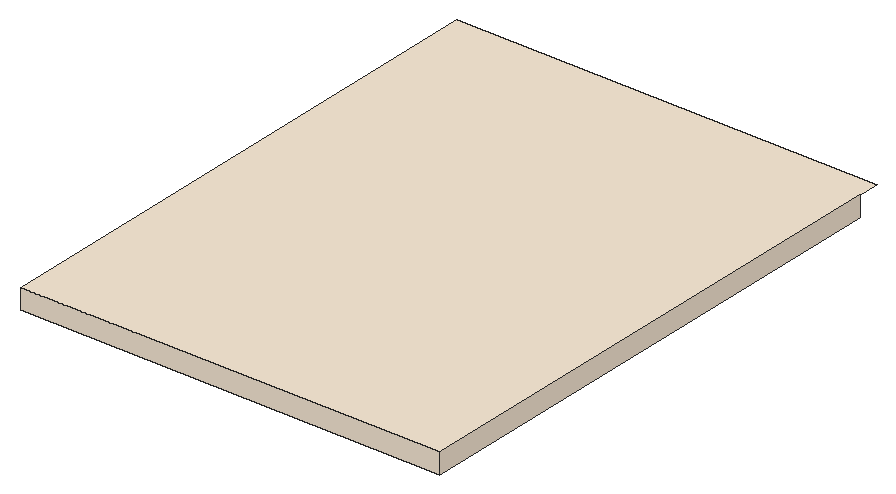
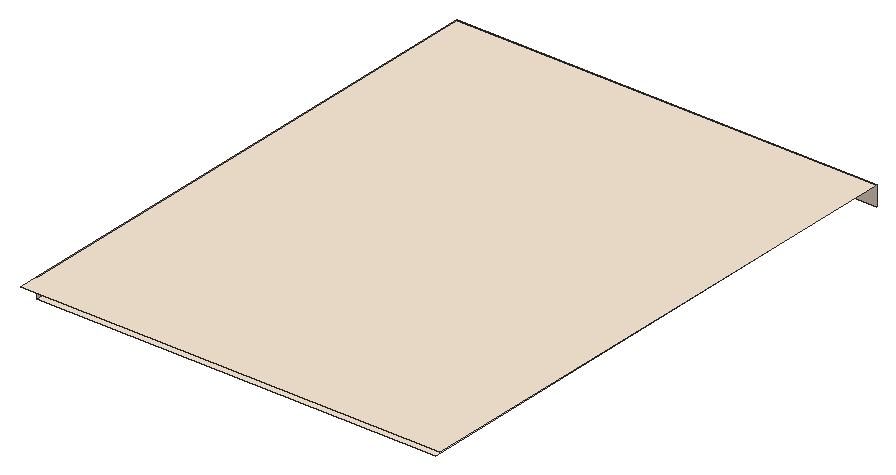
# SketchUp Ruby script. Lengths in inches.
U = 1.inch
M = Sketchup.active_model
def pt(a) = Geom::Point3d.new(a.map { |v| v * U })
def face(e, loops, mat)
  f = e.add_face(loops[0].map { |a| pt(a) })
  loops[1..].each { |l| e.add_face(l.map { |a| pt(a) }).erase! }
  f.material = f.back_material = mat if mat
  f
end
# faces: each face lists its corners as indices into pts; further lists are holes
def faces(e, pts, list, mat = nil) = list.each { |f| face(e, (f[0].is_a?(Array) ? f : [f]).map { |l| l.map { |i| pts[i] } }, mat) }
# xy, xz, yz: faces in a plane at the given z, y or x. An outline is a flat list of corners, or four numbers for a rectangle; further outlines are holes
def ring(l) = l.size == 4 ? [[l[0], l[1]], [l[2], l[1]], [l[2], l[3]], [l[0], l[3]]] : l.each_slice(2).to_a
def flat(e, list, mat, &to3) = list.each { |f| face(e, (f[0].is_a?(Array) ? f : [f]).map { |l| ring(l).map { |u, v| to3.(u, v) } }, mat) }
def xy(e, z, list, mat = nil) = flat(e, list, mat) { |x, y| [x, y, z] }
def xz(e, y, list, mat = nil) = flat(e, list, mat) { |x, z| [x, y, z] }
def yz(e, x, list, mat = nil) = flat(e, list, mat) { |y, z| [x, y, z] }
def lines(e, pts, list) = list.each { |a, b| e.add_line(pt(pts[a]), pt(pts[b])) }
# prism: a flat outline (further loops are holes) pulled along v
def prism(e, loops, v, mat = nil)
  f = face(e, loops, mat); d = Geom::Vector3d.new(v.map { |x| x * U })
  f.pushpull(f.normal.samedirection?(d) ? d.length : -d.length)
end
def box(e, o, s, mat = nil) = prism(e, [[o, [o[0] + s[0], o[1], o[2]], [o[0] + s[0], o[1] + s[1], o[2]], [o[0], o[1] + s[1], o[2]]]], [0, 0, s[2]], mat)
def at(x, y, z, deg = 0) = Geom::Transformation.translation(pt([x, y, z])) * Geom::Transformation.rotation(ORIGIN, Z_AXIS, deg.degrees)
def axes(o, x, y, z) = Geom::Transformation.new([*x, 0, *y, 0, *z, 0, *pt(o).to_a, 1])
def part(name) = M.definitions.add(name)
# library, detail: a bought-in or finely detailed component or shape, given as its bounding box
def library(name, o, s) = part(name).tap { |d| box(d.entities, o, s) }
def detail(e, o, s) = box(e.add_group.entities, o, s)
def put(e, d, t, mat = nil) = e.add_instance(d, t).tap { |i| i.material = mat if mat }
def group(e, t, mat = nil) = e.add_group.tap { |g| g.transformation = t; g.material = mat if mat }.entities
root = M.entities
M.materials.add("[0028_AntiqueWhite]").color = [250, 235, 215]
M.materials.add("[Granite Light Gray]").color = [149, 148, 144]
xy(root,231.4,[[[30.25,60.67,29.63,60.78,29.02,60.95,28.43,61.19,27.87,61.49,27.35,61.84,26.86,62.24,26.41,62.6875,26.01,63.18,25.67,63.71,25.38,64.27,25.15,64.86,24.98,65.47,24.98,232.53,25.03,233.34,25.1875,234.13,25.45,234.9,25.81,235.62,26.25,236.29,26.79,236.9,27.39,237.43,28.07,237.88,28.79,238.24,29.55,238.5,30.35,238.66,31.15,238.71,182.85,238.71,183.6,238.55,184.33,238.3,185.02,237.96,185.67,237.55,186.27,237.0625,186.81,236.51,187.27,235.9,187.66,235.23,187.97,234.53,188.2,233.79,188.33,233.03,188.38,232.26,188.38,66.48,188.2,65.68,187.93,64.92,187.57,64.1875,187.13,63.5,186.61,62.875,186.02,62.31,185.37,61.83,184.67,61.42,183.92,61.09,183.14,60.86,182.34,60.71,181.53,60.67],[30.47,63.11,181.46,63.11,182.06,63.14,182.58,63.24,183.08,63.39,183.5625,63.6,184.02,63.86,184.4375,64.18,184.82,64.54,185.15,64.95,185.44,65.39,185.67,65.86,185.85,66.36,185.93,66.75,185.93,232.19,185.9,232.74,185.82,233.22,185.68,233.68,185.48,234.12,185.24,234.53,184.95,234.92,184.61,235.26,184.24,235.57,183.83,235.82,183.4,236.03,182.95,236.1875,182.59,236.27,31.15,236.27,30.67,236.23,30.1875,236.14,29.72,235.98,29.29,235.77,28.88,235.49,28.51,235.17,28.19,234.81,27.92,234.4,27.71,233.96,27.55,233.5,27.45,233.02,27.42,232.53,27.42,65.81,27.47,65.64,27.61,65.28,27.78,64.9375,27.99,64.62,28.23,64.32,28.5,64.05,28.8,63.8,29.12,63.59,29.46,63.41,29.82,63.27,30.1875,63.16]]],"[Granite Light Gray]")
xy(root,232.34,[[[37.8125,67.21,37.07,67.33,36.34,67.53,35.63,67.81,34.96,68.15,34.33,68.57,33.74,69.04,33.21,69.58,32.74,70.17,32.33,70.8,31.99,71.48,31.72,72.18,31.52,72.91,31.52,227.33,31.66,227.92,31.86,228.49,32.12,229.04,32.42,229.5625,32.78,230.05,33.19,230.5,33.64,230.9,34.125,231.26,34.65,231.57,35.2,231.83,35.77,232.02,36.36,232.16,177.3125,232.16,177.86,232.03,178.4,231.85,178.91,231.61,179.4,231.33,179.86,230.99,180.28,230.61,180.66,230.19,181,229.73,181.28,229.25,181.52,228.73,181.7,228.19,181.83,227.64,181.83,71.75,181.71,71.13,181.51,70.53,181.24,69.97,180.91,69.43,180.52,68.94,180.07,68.5,179.57,68.12,179.03,67.8,178.46,67.54,177.86,67.36,177.24,67.25,176.61,67.21],[37.91,68.4,176.58,68.4,177.1,68.43,177.58,68.52,178.04,68.66,178.49,68.86,178.9,69.11,179.29,69.4,179.64,69.74,179.94,70.12,180.2,70.53,180.4,70.97,180.56,71.4375,180.64,71.87,180.64,227.51,180.56,227.87,180.41,228.29,180.23,228.69,180,229.08,179.74,229.4375,179.4375,229.77,179.11,230.07,178.75,230.33,178.36,230.56,177.96,230.75,177.53,230.89,177.18,230.97,36.5,230.97,36.1,230.88,35.64,230.72,35.2,230.52,34.78,230.27,34.39,229.98,34.03,229.66,33.71,229.3,33.42,228.9,33.17,228.49,32.97,228.04,32.81,227.59,32.71,227.19,32.71,73.07,32.85,72.55,33.08,71.96,33.36,71.4,33.7,70.87,34.1,70.375,34.54,69.93,35.03,69.53,35.5625,69.18,36.12,68.89,36.71,68.66,37.32,68.5]]],"[Granite Light Gray]")
xy(root,233.77,[[24.97,7.66,24.05,7.72,23.14,7.9,22.26,8.2,21.43,8.61,20.66,9.12,19.96,9.73,19.35,10.43,18.84,11.2,18.43,12.03,18.13,12.91,17.95,13.82,17.89,14.74,17.89,31.67,17.94,32.53,18.11,33.38,18.39,34.2,18.77,34.97,19.25,35.69,19.82,36.33,20.47,36.9,21.18,37.38,21.95,37.76,22.77,38.04,23.62,38.21,24.48,38.26,190.49,38.26,191.11,38.14,191.71,37.96,192.29,37.71,192.84,37.4,193.35,37.03,193.82,36.61,194.24,36.14,194.61,35.63,194.92,35.08,195.16,34.5,195.35,33.9,195.47,33.28,195.47,12.37,195.34,11.73,195.14,11.11,194.86,10.52,194.52,9.97,194.11,9.46,193.64,9,193.125,8.6,192.5625,8.27,191.97,8,191.34,7.8125,190.7,7.7,190.05,7.66]],"[Granite Light Gray]")
xy(root,234.21,[[[10.23,45.92,203.125,253.46],[30.25,60.67,181.53,60.67,182.34,60.71,183.14,60.86,183.92,61.09,184.67,61.42,185.37,61.83,186.02,62.31,186.61,62.875,187.13,63.5,187.57,64.1875,187.93,64.92,188.2,65.68,188.38,66.48,188.38,232.26,188.33,233.03,188.2,233.79,187.97,234.53,187.66,235.23,187.27,235.9,186.81,236.51,186.27,237.0625,185.67,237.55,185.02,237.96,184.33,238.3,183.6,238.55,182.85,238.71,31.15,238.71,30.35,238.66,29.55,238.5,28.79,238.24,28.07,237.88,27.39,237.43,26.79,236.9,26.25,236.29,25.81,235.62,25.45,234.9,25.1875,234.13,25.03,233.34,24.98,232.53,24.98,65.47,25.15,64.86,25.38,64.27,25.67,63.71,26.01,63.18,26.41,62.6875,26.86,62.24,27.35,61.84,27.87,61.49,28.43,61.19,29.02,60.95,29.63,60.78]],[37.91,68.4,37.32,68.5,36.71,68.66,36.12,68.89,35.5625,69.18,35.03,69.53,34.54,69.93,34.1,70.375,33.7,70.87,33.36,71.4,33.08,71.96,32.85,72.55,32.71,73.07,32.71,227.19,32.81,227.59,32.97,228.04,33.17,228.49,33.42,228.9,33.71,229.3,34.03,229.66,34.39,229.98,34.78,230.27,35.2,230.52,35.64,230.72,36.1,230.88,36.5,230.97,177.18,230.97,177.53,230.89,177.96,230.75,178.36,230.56,178.75,230.33,179.11,230.07,179.4375,229.77,179.74,229.4375,180,229.08,180.23,228.69,180.41,228.29,180.56,227.87,180.64,227.51,180.64,71.87,180.56,71.4375,180.4,70.97,180.2,70.53,179.94,70.12,179.64,69.74,179.29,69.4,178.9,69.11,178.49,68.86,178.04,68.66,177.58,68.52,177.1,68.43,176.58,68.4]],"[0028_AntiqueWhite]")
xy(root,234.21,[[[30.47,63.11,30.1875,63.16,29.82,63.27,29.46,63.41,29.12,63.59,28.8,63.8,28.5,64.05,28.23,64.32,27.99,64.62,27.78,64.9375,27.61,65.28,27.47,65.64,27.42,65.81,27.42,232.53,27.45,233.02,27.55,233.5,27.71,233.96,27.92,234.4,28.19,234.81,28.51,235.17,28.88,235.49,29.29,235.77,29.72,235.98,30.1875,236.14,30.67,236.23,31.15,236.27,182.59,236.27,182.95,236.1875,183.4,236.03,183.83,235.82,184.24,235.57,184.61,235.26,184.95,234.92,185.24,234.53,185.48,234.12,185.68,233.68,185.82,233.22,185.9,232.74,185.93,232.19,185.93,66.75,185.85,66.36,185.67,65.86,185.44,65.39,185.15,64.95,184.82,64.54,184.4375,64.18,184.02,63.86,183.5625,63.6,183.08,63.39,182.58,63.24,182.06,63.14,181.46,63.11],[37.8125,67.21,176.61,67.21,177.24,67.25,177.86,67.36,178.46,67.54,179.03,67.8,179.57,68.12,180.07,68.5,180.52,68.94,180.91,69.43,181.24,69.97,181.51,70.53,181.71,71.13,181.83,71.75,181.83,227.64,181.7,228.19,181.52,228.73,181.28,229.25,181,229.73,180.66,230.19,180.28,230.61,179.86,230.99,179.4,231.33,178.91,231.61,178.4,231.85,177.86,232.03,177.3125,232.16,36.36,232.16,35.77,232.02,35.2,231.83,34.65,231.57,34.125,231.26,33.64,230.9,33.19,230.5,32.78,230.05,32.42,229.5625,32.12,229.04,31.86,228.49,31.66,227.92,31.52,227.33,31.52,72.91,31.72,72.18,31.99,71.48,32.33,70.8,32.74,70.17,33.21,69.58,33.74,69.04,34.33,68.57,34.96,68.15,35.63,67.81,36.34,67.53,37.07,67.33]]],"[Granite Light Gray]")
xy(root,243.9,[[0,0,203.125,263.6875]],"[0028_AntiqueWhite]")
xz(root,0,[[0,234.21,203.125,243.9]],"[0028_AntiqueWhite]")
xz(root,60.67,[[30.25,231.4,181.53,234.21]],"[Granite Light Gray]")
xz(root,63.11,[[30.47,231.4,181.46,234.21]],"[Granite Light Gray]")
xz(root,67.21,[[37.8125,232.34,176.61,234.21]],"[0028_AntiqueWhite]")
xz(root,68.4,[[37.91,232.34,176.58,234.21]],"[Granite Light Gray]")
xz(root,230.97,[[36.5,232.34,177.18,234.21]],"[Granite Light Gray]")
xz(root,232.16,[[36.36,232.34,177.3125,234.21]],"[Granite Light Gray]")
xz(root,236.27,[[31.15,231.4,182.59,234.21]],"[Granite Light Gray]")
xz(root,238.71,[[31.15,231.4,182.85,234.21]],"[Granite Light Gray]")
yz(root,24.98,[[65.47,231.4,232.53,234.21]],"[0028_AntiqueWhite]")
yz(root,27.42,[[65.81,231.4,232.53,234.21]],"[Granite Light Gray]")
yz(root,31.52,[[72.91,232.34,227.33,234.21]],"[0028_AntiqueWhite]")
yz(root,32.71,[[73.07,232.34,227.19,234.21]],"[Granite Light Gray]")
yz(root,180.64,[[71.87,232.34,227.51,234.21]],"[0028_AntiqueWhite]")
yz(root,181.83,[[71.75,232.34,227.64,234.21]],"[Granite Light Gray]")
yz(root,185.93,[[66.75,231.4,232.19,234.21]],"[0028_AntiqueWhite]")
yz(root,188.38,[[66.48,231.4,232.26,234.21]],"[Granite Light Gray]")
yz(root,203.125,[[0,234.21,253.46,243.9]],"[0028_AntiqueWhite]")
p = [[30.25,60.67,234.21],[29.63,60.78,234.21],[29.63,60.78,231.4],[30.25,60.67,231.4],[182.34,60.71,234.21],[181.53,60.67,234.21],
  [181.53,60.67,231.4],[182.34,60.71,231.4],[183.14,60.86,234.21],[183.14,60.86,231.4],[29.02,60.95,234.21],[29.02,60.95,231.4],
  [183.92,61.09,234.21],[183.92,61.09,231.4],[28.43,61.19,234.21],[28.43,61.19,231.4],[184.67,61.42,234.21],[184.67,61.42,231.4],
  [27.87,61.49,234.21],[27.87,61.49,231.4],[185.37,61.83,234.21],[185.37,61.83,231.4],[27.35,61.84,234.21],[27.35,61.84,231.4],
  [26.86,62.24,234.21],[26.86,62.24,231.4],[186.02,62.31,234.21],[186.02,62.31,231.4],[26.41,62.6875,234.21],[26.41,62.6875,231.4],
  [186.61,62.875,234.21],[186.61,62.875,231.4],[26.01,63.18,234.21],[26.01,63.18,231.4],[187.13,63.5,234.21],[187.13,63.5,231.4],
  [30.1875,63.16,234.21],[30.47,63.11,234.21],[30.47,63.11,231.4],[30.1875,63.16,231.4],[181.46,63.11,234.21],[182.06,63.14,234.21],
  [182.06,63.14,231.4],[181.46,63.11,231.4],[182.58,63.24,234.21],[182.58,63.24,231.4],[25.67,63.71,234.21],[25.67,63.71,231.4],
  [29.82,63.27,234.21],[29.82,63.27,231.4],[183.08,63.39,234.21],[183.08,63.39,231.4],[29.46,63.41,234.21],[29.46,63.41,231.4],
  [29.12,63.59,234.21],[29.12,63.59,231.4],[183.5625,63.6,234.21],[183.5625,63.6,231.4],[187.57,64.1875,234.21],[187.57,64.1875,231.4],
  [28.8,63.8,234.21],[28.8,63.8,231.4],[184.02,63.86,234.21],[184.02,63.86,231.4],[25.38,64.27,234.21],[25.38,64.27,231.4],
  [28.5,64.05,234.21],[28.5,64.05,231.4],[184.4375,64.18,234.21],[184.4375,64.18,231.4],[28.23,64.32,234.21],[28.23,64.32,231.4],
  [184.82,64.54,234.21],[184.82,64.54,231.4],[187.93,64.92,234.21],[187.93,64.92,231.4],[25.15,64.86,234.21],[25.15,64.86,231.4],
  [27.99,64.62,234.21],[27.99,64.62,231.4],[185.15,64.95,234.21],[185.15,64.95,231.4],[27.78,64.9375,234.21],[27.78,64.9375,231.4],
  [24.98,65.47,234.21],[24.98,65.47,231.4],[27.61,65.28,234.21],[27.61,65.28,231.4],[185.44,65.39,234.21],[185.44,65.39,231.4],
  [188.2,65.68,234.21],[188.2,65.68,231.4],[27.47,65.64,234.21],[27.47,65.64,231.4],[185.67,65.86,234.21],[185.67,65.86,231.4],
  [27.42,65.81,234.21],[27.42,65.81,231.4],[188.38,66.48,234.21],[188.38,66.48,231.4],[185.85,66.36,234.21],[185.85,66.36,231.4],
  [185.93,66.75,234.21],[185.93,66.75,231.4],[185.93,232.19,234.21],[185.9,232.74,234.21],[185.9,232.74,231.4],[185.93,232.19,231.4],
  [188.33,233.03,234.21],[188.38,232.26,234.21],[188.38,232.26,231.4],[188.33,233.03,231.4],[24.98,232.53,234.21],[25.03,233.34,234.21],
  [25.03,233.34,231.4],[24.98,232.53,231.4],[27.45,233.02,234.21],[27.42,232.53,234.21],[27.42,232.53,231.4],[27.45,233.02,231.4],
  [185.82,233.22,234.21],[185.82,233.22,231.4],[27.55,233.5,234.21],[27.55,233.5,231.4],[188.2,233.79,234.21],[188.2,233.79,231.4],
  [185.68,233.68,234.21],[185.68,233.68,231.4],[25.1875,234.13,234.21],[25.1875,234.13,231.4],[27.71,233.96,234.21],[27.71,233.96,231.4],
  [185.48,234.12,234.21],[185.48,234.12,231.4],[187.97,234.53,234.21],[187.97,234.53,231.4],[27.92,234.4,234.21],[27.92,234.4,231.4],
  [25.45,234.9,234.21],[25.45,234.9,231.4],[185.24,234.53,234.21],[185.24,234.53,231.4],[28.19,234.81,234.21],[28.19,234.81,231.4],
  [184.95,234.92,234.21],[184.95,234.92,231.4],[187.66,235.23,234.21],[187.66,235.23,231.4],[28.51,235.17,234.21],[28.51,235.17,231.4],
  [25.81,235.62,234.21],[25.81,235.62,231.4],[184.61,235.26,234.21],[184.61,235.26,231.4],[28.88,235.49,234.21],[28.88,235.49,231.4],
  [187.27,235.9,234.21],[187.27,235.9,231.4],[184.24,235.57,234.21],[184.24,235.57,231.4],[29.29,235.77,234.21],[29.29,235.77,231.4],
  [26.25,236.29,234.21],[26.25,236.29,231.4],[183.83,235.82,234.21],[183.83,235.82,231.4],[29.72,235.98,234.21],[29.72,235.98,231.4],
  [183.4,236.03,234.21],[183.4,236.03,231.4],[186.81,236.51,234.21],[186.81,236.51,231.4],[30.1875,236.14,234.21],[30.1875,236.14,231.4],
  [182.95,236.1875,234.21],[182.95,236.1875,231.4],[30.67,236.23,234.21],[30.67,236.23,231.4],[31.15,236.27,234.21],[31.15,236.27,231.4],
  [182.59,236.27,234.21],[182.59,236.27,231.4],[26.79,236.9,234.21],[26.79,236.9,231.4],[186.27,237.0625,234.21],[186.27,237.0625,231.4],
  [27.39,237.43,234.21],[27.39,237.43,231.4],[185.67,237.55,234.21],[185.67,237.55,231.4],[28.07,237.88,234.21],[28.07,237.88,231.4],
  [185.02,237.96,234.21],[185.02,237.96,231.4],[28.79,238.24,234.21],[28.79,238.24,231.4],[184.33,238.3,234.21],[184.33,238.3,231.4],
  [29.55,238.5,234.21],[29.55,238.5,231.4],[183.6,238.55,234.21],[183.6,238.55,231.4],[30.35,238.66,234.21],[30.35,238.66,231.4],
  [182.85,238.71,234.21],[182.85,238.71,231.4],[31.15,238.71,234.21],[31.15,238.71,231.4],[37.8125,67.21,234.21],[37.07,67.33,234.21],
  [37.07,67.33,232.34],[37.8125,67.21,232.34],[177.24,67.25,234.21],[176.61,67.21,234.21],[176.61,67.21,232.34],[177.24,67.25,232.34],
  [177.86,67.36,234.21],[177.86,67.36,232.34],[36.34,67.53,234.21],[36.34,67.53,232.34],[178.46,67.54,234.21],[178.46,67.54,232.34],
  [35.63,67.81,234.21],[35.63,67.81,232.34],[179.03,67.8,234.21],[179.03,67.8,232.34],[34.96,68.15,234.21],[34.96,68.15,232.34],
  [179.57,68.12,234.21],[179.57,68.12,232.34],[180.07,68.5,234.21],[180.07,68.5,232.34],[34.33,68.57,234.21],[34.33,68.57,232.34],
  [37.32,68.5,234.21],[37.91,68.4,234.21],[37.91,68.4,232.34],[37.32,68.5,232.34],[176.58,68.4,234.21],[177.1,68.43,234.21],
  [177.1,68.43,232.34],[176.58,68.4,232.34],[177.58,68.52,234.21],[177.58,68.52,232.34],[36.71,68.66,234.21],[36.71,68.66,232.34],
  [178.04,68.66,234.21],[178.04,68.66,232.34],[180.52,68.94,234.21],[180.52,68.94,232.34],[33.74,69.04,234.21],[33.74,69.04,232.34],
  [36.12,68.89,234.21],[36.12,68.89,232.34],[178.49,68.86,234.21],[178.49,68.86,232.34],[35.5625,69.18,234.21],[35.5625,69.18,232.34],
  [178.9,69.11,234.21],[178.9,69.11,232.34],[180.91,69.43,234.21],[180.91,69.43,232.34],[33.21,69.58,234.21],[33.21,69.58,232.34],
  [179.29,69.4,234.21],[179.29,69.4,232.34],[35.03,69.53,234.21],[35.03,69.53,232.34],[179.64,69.74,234.21],[179.64,69.74,232.34],
  [181.24,69.97,234.21],[181.24,69.97,232.34],[34.54,69.93,234.21],[34.54,69.93,232.34],[32.74,70.17,234.21],[32.74,70.17,232.34],
  [179.94,70.12,234.21],[179.94,70.12,232.34],[34.1,70.375,234.21],[34.1,70.375,232.34],[181.51,70.53,234.21],[181.51,70.53,232.34],
  [180.2,70.53,234.21],[180.2,70.53,232.34],[32.33,70.8,234.21],[32.33,70.8,232.34],[33.7,70.87,234.21],[33.7,70.87,232.34],
  [180.4,70.97,234.21],[180.4,70.97,232.34],[181.71,71.13,234.21],[181.71,71.13,232.34],[31.99,71.48,234.21],[31.99,71.48,232.34],
  [33.36,71.4,234.21],[33.36,71.4,232.34],[180.56,71.4375,234.21],[180.56,71.4375,232.34],[181.83,71.75,234.21],[181.83,71.75,232.34],
  [33.08,71.96,234.21],[33.08,71.96,232.34],[180.64,71.87,234.21],[180.64,71.87,232.34],[31.72,72.18,234.21],[31.72,72.18,232.34],
  [32.85,72.55,234.21],[32.85,72.55,232.34],[31.52,72.91,234.21],[31.52,72.91,232.34],[32.71,73.07,234.21],[32.71,73.07,232.34],
  [32.81,227.59,234.21],[32.71,227.19,234.21],[32.71,227.19,232.34],[32.81,227.59,232.34],[31.52,227.33,234.21],[31.66,227.92,234.21],
  [31.66,227.92,232.34],[31.52,227.33,232.34],[180.64,227.51,234.21],[180.56,227.87,234.21],[180.56,227.87,232.34],[180.64,227.51,232.34],
  [32.97,228.04,234.21],[32.97,228.04,232.34],[181.7,228.19,234.21],[181.83,227.64,234.21],[181.83,227.64,232.34],[181.7,228.19,232.34],
  [31.86,228.49,234.21],[31.86,228.49,232.34],[180.41,228.29,234.21],[180.41,228.29,232.34],[33.17,228.49,234.21],[33.17,228.49,232.34],
  [181.52,228.73,234.21],[181.52,228.73,232.34],[180.23,228.69,234.21],[180.23,228.69,232.34],[32.12,229.04,234.21],[32.12,229.04,232.34],
  [33.42,228.9,234.21],[33.42,228.9,232.34],[180,229.08,234.21],[180,229.08,232.34],[181.28,229.25,234.21],[181.28,229.25,232.34],
  [33.71,229.3,234.21],[33.71,229.3,232.34],[32.42,229.5625,234.21],[32.42,229.5625,232.34],[179.74,229.4375,234.21],[179.74,229.4375,232.34],
  [181,229.73,234.21],[181,229.73,232.34],[34.03,229.66,234.21],[34.03,229.66,232.34],[179.4375,229.77,234.21],[179.4375,229.77,232.34],
  [32.78,230.05,234.21],[32.78,230.05,232.34],[34.39,229.98,234.21],[34.39,229.98,232.34],[180.66,230.19,234.21],[180.66,230.19,232.34],
  [179.11,230.07,234.21],[179.11,230.07,232.34],[33.19,230.5,234.21],[33.19,230.5,232.34],[34.78,230.27,234.21],[34.78,230.27,232.34],
  [178.75,230.33,234.21],[178.75,230.33,232.34],[180.28,230.61,234.21],[180.28,230.61,232.34],[35.2,230.52,234.21],[35.2,230.52,232.34],
  [178.36,230.56,234.21],[178.36,230.56,232.34],[33.64,230.9,234.21],[33.64,230.9,232.34],[35.64,230.72,234.21],[35.64,230.72,232.34],
  [177.96,230.75,234.21],[177.96,230.75,232.34],[179.86,230.99,234.21],[179.86,230.99,232.34],[36.1,230.88,234.21],[36.1,230.88,232.34],
  [177.53,230.89,234.21],[177.53,230.89,232.34],[34.125,231.26,234.21],[34.125,231.26,232.34],[36.5,230.97,234.21],[36.5,230.97,232.34],
  [177.18,230.97,234.21],[177.18,230.97,232.34],[179.4,231.33,234.21],[179.4,231.33,232.34],[34.65,231.57,234.21],[34.65,231.57,232.34],
  [178.91,231.61,234.21],[178.91,231.61,232.34],[35.2,231.83,234.21],[35.2,231.83,232.34],[178.4,231.85,234.21],[178.4,231.85,232.34],
  [35.77,232.02,234.21],[35.77,232.02,232.34],[177.86,232.03,234.21],[177.86,232.03,232.34],[36.36,232.16,234.21],[36.36,232.16,232.34],
  [177.3125,232.16,234.21],[177.3125,232.16,232.34],[203.125,0,234.21],[203.125,-0.64,234.21]]
faces(root,p,[[0,1,2,3],[1,10,11,2],[10,14,15,11],[14,18,19,15],[18,22,23,19],[22,24,25,23],[24,28,29,25],[28,32,33,29],
  [40,41,42,43],[41,44,45,42],[32,46,47,33],[44,50,51,45],[50,56,57,51],[56,62,63,57],[46,64,65,47],[62,68,69,63],
  [68,72,73,69],[64,76,77,65],[72,80,81,73],[76,84,85,77],[80,88,89,81],[88,94,95,89],[94,100,101,95],[100,102,103,101],
  [104,105,106,107],[112,113,114,115],[105,120,121,106],[120,126,127,121],[113,128,129,114],[126,132,133,127],[128,138,139,129],[132,140,141,133],
  [140,144,145,141],[138,150,151,139],[144,152,153,145],[152,158,159,153],[150,162,163,151],[158,164,165,159],[164,168,169,165],[168,174,175,169],
  [174,180,181,175],[162,182,183,163],[182,186,187,183],[186,190,191,187],[190,194,195,191],[194,198,199,195],[198,202,203,199],[202,206,207,203],
  [208,209,210,211],[209,218,219,210],[218,222,223,219],[222,226,227,223],[226,232,233,227],[238,239,240,241],[239,242,243,240],[242,246,247,243],
  [232,250,251,233],[246,254,255,247],[254,258,259,255],[250,262,263,251],[258,264,265,259],[264,268,269,265],[262,274,275,263],[268,276,277,269],
  [276,282,283,277],[274,284,285,275],[282,288,289,283],[284,292,293,285],[288,296,297,289],[296,302,303,297],[292,304,305,293],[304,308,309,305],
  [316,317,318,319],[320,321,322,323],[317,330,331,318],[321,332,333,322],[332,338,339,333],[330,340,341,331],[338,344,345,339],[340,350,351,341],
  [344,352,353,345],[352,358,359,353],[350,360,361,351],[358,366,367,359],[360,368,369,361],[366,372,373,367],[372,378,379,373],[368,380,381,369],
  [378,384,385,379],[384,390,391,385],[380,392,393,381],[390,396,397,391],[392,400,401,393],[400,404,405,401],[404,408,409,405],[408,412,413,409]],"[0028_AntiqueWhite]")
faces(root,p,[[4,5,6,7],[8,4,7,9],[12,8,9,13],[16,12,13,17],[20,16,17,21],[26,20,21,27],[30,26,27,31],[34,30,31,35],
  [36,37,38,39],[48,36,39,49],[52,48,49,53],[54,52,53,55],[58,34,35,59],[60,54,55,61],[66,60,61,67],[70,66,67,71],
  [74,58,59,75],[78,70,71,79],[82,78,79,83],[86,82,83,87],[90,74,75,91],[92,86,87,93],[96,92,93,97],[98,90,91,99],
  [108,109,110,111],[116,117,118,119],[122,116,119,123],[124,108,111,125],[130,122,123,131],[134,124,125,135],[136,130,131,137],[142,136,137,143],
  [146,134,135,147],[148,142,143,149],[154,148,149,155],[156,146,147,157],[160,154,155,161],[166,160,161,167],[170,156,157,171],[172,166,167,173],
  [176,172,173,177],[178,176,177,179],[184,170,171,185],[188,184,185,189],[192,188,189,193],[196,192,193,197],[200,196,197,201],[204,200,201,205],
  [212,213,214,215],[216,212,215,217],[220,216,217,221],[224,220,221,225],[228,224,225,229],[230,228,229,231],[234,235,236,237],[244,234,237,245],
  [248,230,231,249],[252,244,245,253],[256,252,253,257],[260,248,249,261],[266,256,257,267],[270,260,261,271],[272,266,267,273],[278,272,273,279],
  [280,270,271,281],[286,278,279,287],[290,280,281,291],[294,286,287,295],[298,290,291,299],[300,294,295,301],[306,300,301,307],[310,306,307,311],
  [312,313,314,315],[324,312,315,325],[326,327,328,329],[334,324,325,335],[336,326,329,337],[342,334,335,343],[346,336,337,347],[348,342,343,349],
  [354,346,347,355],[356,348,349,357],[362,356,357,363],[364,354,355,365],[370,362,363,371],[374,364,365,375],[376,370,371,377],[382,376,377,383],
  [386,374,375,387],[388,382,383,389],[394,388,389,395],[398,386,387,399],[402,398,399,403],[406,402,403,407],[410,406,407,411],[414,410,411,415]],"[Granite Light Gray]")
lines(root,p,[[416,417]])
